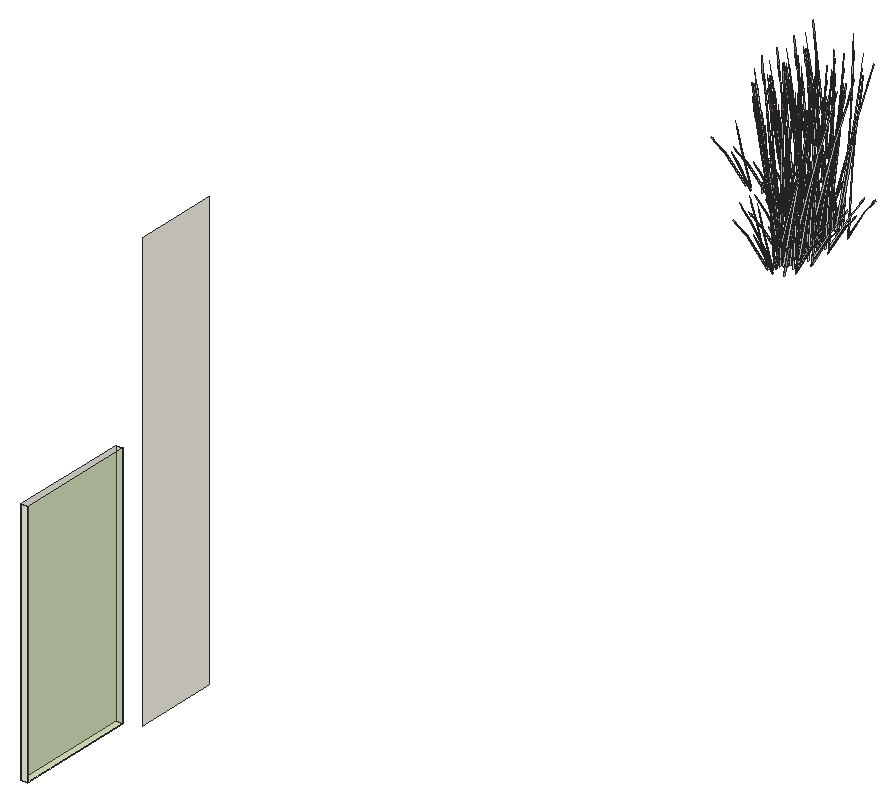
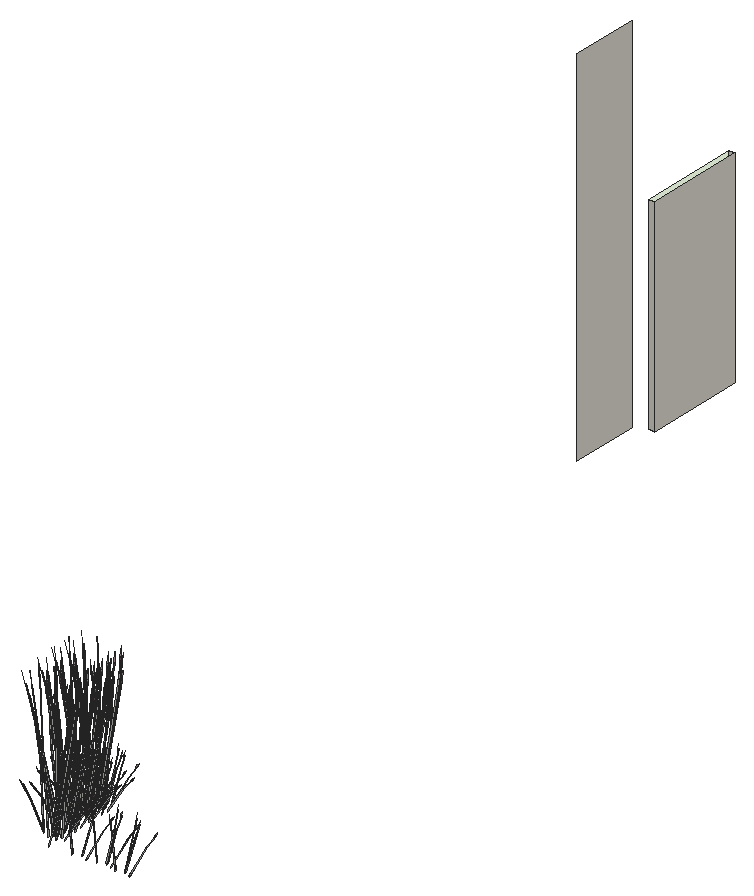
# SketchUp Ruby script. Lengths in inches.
U = 1.inch
M = Sketchup.active_model
def pt(a) = Geom::Point3d.new(a.map { |v| v * U })
def face(e, loops, mat)
  f = e.add_face(loops[0].map { |a| pt(a) })
  loops[1..].each { |l| e.add_face(l.map { |a| pt(a) }).erase! }
  f.material = f.back_material = mat if mat
  f
end
# faces: each face lists its corners as indices into pts; further lists are holes
def faces(e, pts, list, mat = nil) = list.each { |f| face(e, (f[0].is_a?(Array) ? f : [f]).map { |l| l.map { |i| pts[i] } }, mat) }
# xy, xz, yz: faces in a plane at the given z, y or x. An outline is a flat list of corners, or four numbers for a rectangle; further outlines are holes
def ring(l) = l.size == 4 ? [[l[0], l[1]], [l[2], l[1]], [l[2], l[3]], [l[0], l[3]]] : l.each_slice(2).to_a
def flat(e, list, mat, &to3) = list.each { |f| face(e, (f[0].is_a?(Array) ? f : [f]).map { |l| ring(l).map { |u, v| to3.(u, v) } }, mat) }
def xy(e, z, list, mat = nil) = flat(e, list, mat) { |x, y| [x, y, z] }
def xz(e, y, list, mat = nil) = flat(e, list, mat) { |x, z| [x, y, z] }
def yz(e, x, list, mat = nil) = flat(e, list, mat) { |y, z| [x, y, z] }
def lines(e, pts, list) = list.each { |a, b| e.add_line(pt(pts[a]), pt(pts[b])) }
# prism: a flat outline (further loops are holes) pulled along v
def prism(e, loops, v, mat = nil)
  f = face(e, loops, mat); d = Geom::Vector3d.new(v.map { |x| x * U })
  f.pushpull(f.normal.samedirection?(d) ? d.length : -d.length)
end
def box(e, o, s, mat = nil) = prism(e, [[o, [o[0] + s[0], o[1], o[2]], [o[0] + s[0], o[1] + s[1], o[2]], [o[0], o[1] + s[1], o[2]]]], [0, 0, s[2]], mat)
def at(x, y, z, deg = 0) = Geom::Transformation.translation(pt([x, y, z])) * Geom::Transformation.rotation(ORIGIN, Z_AXIS, deg.degrees)
def axes(o, x, y, z) = Geom::Transformation.new([*x, 0, *y, 0, *z, 0, *pt(o).to_a, 1])
def part(name) = M.definitions.add(name)
# library, detail: a bought-in or finely detailed component or shape, given as its bounding box
def library(name, o, s) = part(name).tap { |d| box(d.entities, o, s) }
def detail(e, o, s) = box(e.add_group.entities, o, s)
def put(e, d, t, mat = nil) = e.add_instance(d, t).tap { |i| i.material = mat if mat }
def group(e, t, mat = nil) = e.add_group.tap { |g| g.transformation = t; g.material = mat if mat }.entities
root = M.entities
M.materials.add("C01_Vanilla_Cream").color = [255, 251, 241]
M.materials.add("Glass_Basic_01").color = [119, 186, 61]
M.materials["Glass_Basic_01"].alpha = 0.25
M.materials.add("LightPink_Translucent").color = [144, 107, 117]
M.materials["LightPink_Translucent"].alpha = 0.75
c1 = part("blade")
p = [[2.15,0.21,22],[0,0.17,0],[0.09,0.45,0],[2.18,0.31,22],[2.29,0.31,22],[0.38,0.45,0],
  [2.48,0.24,33],[2.49,0.24,33],[2.48,0.22,33]]
faces(c1.entities,p,[[0,1,2,3],[4,5,2,3],[6,3,4,7],[8,0,3,6]])
c2 = part("seeds")
p = [[0.3,-0.1,1.38],[-0.01,-0.03,1.59],[-0.01,-0.03,0.03],[0.14,-0.07,-0.07],[0.29,-0.03,3],[0.15,0.01,3.11]]
faces(c2.entities,p,[[0,1,2,3],[1,0,4,5]],"LightPink_Translucent")
c3 = part("blade with seeds")
put(c3.entities,c1,at(0,0,0))
put(c3.entities,c2,axes([2.4,0.25,30.99],[1.5799,-0.05474,1.17369],[-0.12525,1.92788,0.29478],[-0.07173,-0.02425,1.56792]))
xy(root,265,[[700,25,702,59]],"C01_Vanilla_Cream")
xz(root,25,[[700,265,702,335]],"C01_Vanilla_Cream")
xz(root,59,[[700,265,702,335]],"C01_Vanilla_Cream")
yz(root,700,[[25,265,59,335]],"C01_Vanilla_Cream")
yz(root,702,[[25,265,59,335]],"Glass_Basic_01")
yz(root,706,[[61,265,84.38,389]],"C01_Vanilla_Cream")
put(root,c3,axes([687.53,307.45,265.24],[-0.10912,0.02057,1.46364],[-0.60346,-0.23156,-0.2236],[0.01013,-0.19315,0.24931]))
put(root,c3,axes([685.57,308.15,265.24],[-0.06302,0.07522,1.46364],[-0.63686,0.16217,-0.2236],[-0.15385,-0.14752,0.24931]))
put(root,c3,axes([690.2,308.43,265.24],[-0.09738,-0.04498,1.46364],[-0.25012,-0.50252,-0.2236],[0.16873,-0.13637,0.24931]))
put(root,c3,axes([687.41,307.85,265.77],[-0.44958,0.32756,-0.03231],[-0.41194,-0.35875,-0.14649],[-0.029,-0.10165,0.48318]))
put(root,c3,axes([687.03,310.37,265.83],[0.31565,-0.51449,-0.37133],[0.65588,0.24761,0.17871],[0,-0.1186,1.19224]))
put(root,c3,axes([687.32,310.12,266.21],[-0.07581,-0.65151,-0.24149],[0.7896,-0.03939,-0.41502],[0.13904,-0.08678,1.32557]))
put(root,c3,axes([685.36,310.15,265.68],[0.45414,-0.35624,-0.25712],[0.45414,0.35624,0.25712],[0,-0.11474,1.15348]))
put(root,c3,axes([685.18,308.44,265.77],[-0.18768,0.46622,-0.03231],[-0.57763,-0.14342,-0.14649],[-0.0877,-0.07626,0.48318]))
put(root,c3,axes([686.95,310.8,266.21],[-0.73268,-0.27244,-0.24149],[0.35279,-0.57501,-0.41502],[-0.02303,-0.14118,1.32557]))
put(root,c3,axes([687.22,308.67,265.68],[0.60696,0.14127,-0.25712],[-0.15283,0.49751,0.25712],[0.12236,-0.05737,1.15348]))
put(root,c3,axes([687.14,311.4,266.02],[0.17244,-0.67657,-0.19446],[0.81759,0.11793,0.42555],[-0.14286,-0.09343,1.29846]))
put(root,c3,axes([687.95,312.39,265.24],[-0.10912,0.02057,1.46364],[-0.60346,-0.23156,-0.2236],[0.01013,-0.19315,0.24931]))
put(root,c3,axes([687.08,311.13,265.83],[-0.39083,-0.47924,-0.37133],[0.59199,-0.33747,0.17871],[-0.12647,-0.0593,1.19224]))
put(root,c3,axes([691.88,310.46,265.875],[-0.40335,-0.3651,-0.05385],[0.44175,-0.33453,-0.24415],[0.12517,-0.02355,0.8053]))
put(root,c3,axes([686.57,309.7,265.32],[-0.64037,0.22859,1.07011],[-0.20382,-0.65589,0.4158],[0.39323,0.01091,1.21713]))
put(root,c3,axes([691.57,310.59,265.24],[-0.034,-0.08668,1.46364],[0.23582,-0.50706,-0.2236],[0.23788,-0.00729,0.24931]))
put(root,c3,axes([684.55,310.5,265.24],[0.0165,0.08998,1.46364],[-0.33262,0.46992,-0.2236],[-0.23626,-0.02369,0.24931]))
put(root,c3,axes([686.01,312.19,265.68],[-0.15283,-0.49751,-0.25712],[0.60696,-0.14127,0.25712],[-0.12236,-0.05737,1.15348]))
put(root,c3,axes([686,313.1,265.24],[-0.06302,0.07522,1.46364],[-0.63686,0.16217,-0.2236],[-0.15385,-0.14752,0.24931]))
put(root,c3,axes([688.23,310.03,266.21],[0.65687,-0.37907,-0.24149],[0.43681,0.53562,-0.41502],[0.16207,0.0544,1.32557]))
put(root,c3,axes([690.62,313.375,265.24],[-0.09738,-0.04498,1.46364],[-0.25012,-0.50252,-0.2236],[0.16873,-0.13637,0.24931]))
put(root,c3,axes([687.5,311.4,266.21],[-0.65687,0.37907,-0.24149],[-0.43681,-0.53562,-0.41502],[-0.16207,-0.0544,1.32557]))
put(root,c3,axes([689.72,309.24,265.68],[0.15283,0.49751,-0.25712],[-0.60696,0.14127,0.25712],[0.12236,0.05737,1.15348]))
put(root,c3,axes([687.84,312.79,265.77],[-0.44958,0.32756,-0.03231],[-0.41194,-0.35875,-0.14649],[-0.029,-0.10165,0.48318]))
put(root,c3,axes([688.63,311.96,265.8125],[0.68303,-0.19373,-0.15934],[0.24001,0.55805,0.00007],[0.07539,-0.02141,1.44335]))
put(root,c3,axes([688.24,311.57,266.05],[-0.63528,-0.45956,-0.20909],[0.53456,-0.51604,0.45758],[-0.17107,0.05376,1.39619]))
put(root,c3,axes([688.65,310.3,265.83],[0.39083,0.47924,-0.37133],[-0.59199,0.33747,0.17871],[0.12647,0.0593,1.19224]))
put(root,c3,axes([687.45,315.31,265.83],[0.31565,-0.51449,-0.37133],[0.65588,0.24761,0.17871],[0,-0.1186,1.19224]))
put(root,c3,axes([687.91,311.47,265.83],[-0.70648,0.03525,-0.37133],[-0.06389,-0.58508,0.17871],[-0.12647,0.0593,1.19224]))
put(root,c3,axes([687.74,315.06,266.21],[-0.07581,-0.65151,-0.24149],[0.7896,-0.03939,-0.41502],[0.13904,-0.08678,1.32557]))
put(root,c3,axes([685.79,315.09,265.68],[0.45414,-0.35624,-0.25712],[0.45414,0.35624,0.25712],[0,-0.11474,1.15348]))
put(root,c3,axes([685.6,313.39,265.77],[-0.18768,0.46622,-0.03231],[-0.57763,-0.14342,-0.14649],[-0.0877,-0.07626,0.48318]))
put(root,c3,axes([687.375,315.74,266.21],[-0.73268,-0.27244,-0.24149],[0.35279,-0.57501,-0.41502],[-0.02303,-0.14118,1.32557]))
put(root,c3,axes([687.64,313.62,265.68],[0.60696,0.14127,-0.25712],[-0.15283,0.49751,0.25712],[0.12236,-0.05737,1.15348]))
put(root,c3,axes([688.51,312.76,265.68],[-0.60696,-0.14127,-0.25712],[0.15283,-0.49751,0.25712],[-0.12236,0.05737,1.15348]))
put(root,c3,axes([688.78,310.63,266.21],[0.73268,0.27244,-0.24149],[-0.35279,0.57501,-0.41502],[0.02303,0.14118,1.32557]))
put(root,c3,axes([687.5625,316.35,266.02],[0.17244,-0.67657,-0.19446],[0.81759,0.11793,0.42555],[-0.14286,-0.09343,1.29846]))
put(root,c3,axes([690.37,311.28,265.68],[-0.45414,0.35624,-0.25712],[-0.45414,-0.35624,0.25712],[0,0.11474,1.15348]))
put(root,c3,axes([688.41,311.32,266.21],[0.07581,0.65151,-0.24149],[-0.7896,0.03939,-0.41502],[-0.13904,0.08678,1.32557]))
put(root,c3,axes([688.7,311.0625,265.83],[-0.31565,0.51449,-0.37133],[-0.65588,-0.24761,0.17871],[0,0.1186,1.19224]))
put(root,c3,axes([687.5,316.07,265.83],[-0.39083,-0.47924,-0.37133],[0.59199,-0.33747,0.17871],[-0.12647,-0.0593,1.19224]))
put(root,c3,axes([692.3,315.4,265.875],[-0.40335,-0.3651,-0.05385],[0.44175,-0.33453,-0.24415],[0.12517,-0.02355,0.8053]))
put(root,c3,axes([687,314.64,265.32],[-0.64037,0.22859,1.07011],[-0.20382,-0.65589,0.4158],[0.39323,0.01091,1.21713]))
put(root,c3,axes([692,315.53,265.24],[-0.034,-0.08668,1.46364],[0.23582,-0.50706,-0.2236],[0.23788,-0.00729,0.24931]))
put(root,c3,axes([689.86,313.09,265.24],[0.0474,-0.08243,1.46364],[0.59674,-0.24277,-0.2236],[0.18092,0.12565,0.24931]))
put(root,c3,axes([684.98,315.44,265.24],[0.0165,0.08998,1.46364],[-0.33262,0.46992,-0.2236],[-0.23626,-0.02369,0.24931]))
put(root,c3,axes([684.375,313.02,265.24],[0.08727,0.05704,1.46364],[0.14797,0.52853,-0.2236],[-0.19341,0.11271,0.24931]))
put(root,c3,axes([686.43,317.14,265.68],[-0.15283,-0.49751,-0.25712],[0.60696,-0.14127,0.25712],[-0.12236,-0.05737,1.15348]))
put(root,c3,axes([687.49,318.93,265.24],[-0.10912,0.02057,1.46364],[-0.60346,-0.23156,-0.2236],[0.01013,-0.19315,0.24931]))
put(root,c3,axes([688.65,314.98,266.21],[0.65687,-0.37907,-0.24149],[0.43681,0.53562,-0.41502],[0.16207,0.0544,1.32557]))
put(root,c3,axes([687.92,316.34,266.21],[-0.65687,0.37907,-0.24149],[-0.43681,-0.53562,-0.41502],[-0.16207,-0.0544,1.32557]))
put(root,c3,axes([690.14,314.18,265.68],[0.15283,0.49751,-0.25712],[-0.60696,0.14127,0.25712],[0.12236,0.05737,1.15348]))
put(root,c3,axes([689.06,316.9,265.8125],[0.68303,-0.19373,-0.15934],[0.24001,0.55805,0.00007],[0.07539,-0.02141,1.44335]))
put(root,c3,axes([687.07,313.07,265.24],[0.10529,-0.03107,1.46364],[0.63335,0.17101,-0.2236],[0.01852,0.19274,0.24931]))
put(root,c3,axes([688.66,316.51,266.05],[-0.63528,-0.45956,-0.20909],[0.53456,-0.51604,0.45758],[-0.17107,0.05376,1.39619]))
put(root,c3,axes([689.07,315.25,265.83],[0.39083,0.47924,-0.37133],[-0.59199,0.33747,0.17871],[0.12647,0.0593,1.19224]))
put(root,c3,axes([685.54,319.64,265.24],[-0.06302,0.07522,1.46364],[-0.63686,0.16217,-0.2236],[-0.15385,-0.14752,0.24931]))
put(root,c3,axes([690.16,319.92,265.24],[-0.09738,-0.04498,1.46364],[-0.25012,-0.50252,-0.2236],[0.16873,-0.13637,0.24931]))
put(root,c3,axes([688.34,316.42,265.83],[-0.70648,0.03525,-0.37133],[-0.06389,-0.58508,0.17871],[-0.12647,0.0593,1.19224]))
put(root,c3,axes([687.38,319.33,265.77],[-0.44958,0.32756,-0.03231],[-0.41194,-0.35875,-0.14649],[-0.029,-0.10165,0.48318]))
put(root,c3,axes([688.9375,317.7,265.68],[-0.60696,-0.14127,-0.25712],[0.15283,-0.49751,0.25712],[-0.12236,0.05737,1.15348]))
put(root,c3,axes([689.2,315.58,266.21],[0.73268,0.27244,-0.24149],[-0.35279,0.57501,-0.41502],[0.02303,0.14118,1.32557]))
put(root,c3,axes([690.79,316.22,265.68],[-0.45414,0.35624,-0.25712],[-0.45414,-0.35624,0.25712],[0,0.11474,1.15348]))
put(root,c3,axes([688.83,316.26,266.21],[0.07581,0.65151,-0.24149],[-0.7896,0.03939,-0.41502],[-0.13904,0.08678,1.32557]))
put(root,c3,axes([689.12,316,265.83],[-0.31565,0.51449,-0.37133],[-0.65588,-0.24761,0.17871],[0,0.1186,1.19224]))
put(root,c3,axes([687.29,321.6,266.21],[-0.07581,-0.65151,-0.24149],[0.7896,-0.03939,-0.41502],[0.13904,-0.08678,1.32557]))
put(root,c3,axes([685.33,321.64,265.68],[0.45414,-0.35624,-0.25712],[0.45414,0.35624,0.25712],[0,-0.11474,1.15348]))
put(root,c3,axes([685.15,319.93,265.77],[-0.18768,0.46622,-0.03231],[-0.57763,-0.14342,-0.14649],[-0.0877,-0.07626,0.48318]))
put(root,c3,axes([686.92,322.28,266.21],[-0.73268,-0.27244,-0.24149],[0.35279,-0.57501,-0.41502],[-0.02303,-0.14118,1.32557]))
put(root,c3,axes([687.18,320.16,265.68],[0.60696,0.14127,-0.25712],[-0.15283,0.49751,0.25712],[0.12236,-0.05737,1.15348]))
put(root,c3,axes([690.28,318.03,265.24],[0.0474,-0.08243,1.46364],[0.59674,-0.24277,-0.2236],[0.18092,0.12565,0.24931]))
put(root,c3,axes([684.8,317.96,265.24],[0.08727,0.05704,1.46364],[0.14797,0.52853,-0.2236],[-0.19341,0.11271,0.24931]))
put(root,c3,axes([687.1,322.89,266.02],[0.17244,-0.67657,-0.19446],[0.81759,0.11793,0.42555],[-0.14286,-0.09343,1.29846]))
put(root,c3,axes([687.05,322.61,265.83],[-0.39083,-0.47924,-0.37133],[0.59199,-0.33747,0.17871],[-0.12647,-0.0593,1.19224]))
put(root,c3,axes([691.85,321.94,265.875],[-0.40335,-0.3651,-0.05385],[0.44175,-0.33453,-0.24415],[0.12517,-0.02355,0.8053]))
put(root,c3,axes([687.49,318.01,265.24],[0.10529,-0.03107,1.46364],[0.63335,0.17101,-0.2236],[0.01852,0.19274,0.24931]))
put(root,c3,axes([686.54,321.18,265.32],[-0.64037,0.22859,1.07011],[-0.20382,-0.65589,0.4158],[0.39323,0.01091,1.21713]))
put(root,c3,axes([691.54,322.07,265.24],[-0.034,-0.08668,1.46364],[0.23582,-0.50706,-0.2236],[0.23788,-0.00729,0.24931]))
put(root,c3,axes([684.52,321.98,265.24],[0.0165,0.08998,1.46364],[-0.33262,0.46992,-0.2236],[-0.23626,-0.02369,0.24931]))
put(root,c3,axes([685.98,323.68,265.68],[-0.15283,-0.49751,-0.25712],[0.60696,-0.14127,0.25712],[-0.12236,-0.05737,1.15348]))
put(root,c3,axes([688.2,321.52,266.21],[0.65687,-0.37907,-0.24149],[0.43681,0.53562,-0.41502],[0.16207,0.0544,1.32557]))
put(root,c3,axes([687.46,322.88,266.21],[-0.65687,0.37907,-0.24149],[-0.43681,-0.53562,-0.41502],[-0.16207,-0.0544,1.32557]))
put(root,c3,axes([689.68,320.72,265.68],[0.15283,0.49751,-0.25712],[-0.60696,0.14127,0.25712],[0.12236,0.05737,1.15348]))
put(root,c3,axes([688.6,323.45,265.8125],[0.68303,-0.19373,-0.15934],[0.24001,0.55805,0.00007],[0.07539,-0.02141,1.44335]))
put(root,c3,axes([688.2,323.06,266.05],[-0.63528,-0.45956,-0.20909],[0.53456,-0.51604,0.45758],[-0.17107,0.05376,1.39619]))
put(root,c3,axes([686.4375,327.13,265.24],[-0.10912,0.02057,1.46364],[-0.60346,-0.23156,-0.2236],[0.01013,-0.19315,0.24931]))
put(root,c3,axes([688.61,321.79,265.83],[0.39083,0.47924,-0.37133],[-0.59199,0.33747,0.17871],[0.12647,0.0593,1.19224]))
put(root,c3,axes([687.88,322.96,265.83],[-0.70648,0.03525,-0.37133],[-0.06389,-0.58508,0.17871],[-0.12647,0.0593,1.19224]))
put(root,c3,axes([688.48,324.24,265.68],[-0.60696,-0.14127,-0.25712],[0.15283,-0.49751,0.25712],[-0.12236,0.05737,1.15348]))
put(root,c3,axes([688.74,322.12,266.21],[0.73268,0.27244,-0.24149],[-0.35279,0.57501,-0.41502],[0.02303,0.14118,1.32557]))
put(root,c3,axes([690.33,322.76,265.68],[-0.45414,0.35624,-0.25712],[-0.45414,-0.35624,0.25712],[0,0.11474,1.15348]))
put(root,c3,axes([684.49,327.84,265.24],[-0.06302,0.07522,1.46364],[-0.63686,0.16217,-0.2236],[-0.15385,-0.14752,0.24931]))
put(root,c3,axes([688.375,322.8,266.21],[0.07581,0.65151,-0.24149],[-0.7896,0.03939,-0.41502],[-0.13904,0.08678,1.32557]))
put(root,c3,axes([688.66,322.54,265.83],[-0.31565,0.51449,-0.37133],[-0.65588,-0.24761,0.17871],[0,0.1186,1.19224]))
put(root,c3,axes([689.11,328.12,265.24],[-0.09738,-0.04498,1.46364],[-0.25012,-0.50252,-0.2236],[0.16873,-0.13637,0.24931]))
put(root,c3,axes([686.33,327.53,265.77],[-0.44958,0.32756,-0.03231],[-0.41194,-0.35875,-0.14649],[-0.029,-0.10165,0.48318]))
put(root,c3,axes([689.82,324.57,265.24],[0.0474,-0.08243,1.46364],[0.59674,-0.24277,-0.2236],[0.18092,0.12565,0.24931]))
put(root,c3,axes([684.34,324.5,265.24],[0.08727,0.05704,1.46364],[0.14797,0.52853,-0.2236],[-0.19341,0.11271,0.24931]))
put(root,c3,axes([686.23,329.8,266.21],[-0.07581,-0.65151,-0.24149],[0.7896,-0.03939,-0.41502],[0.13904,-0.08678,1.32557]))
put(root,c3,axes([684.27,329.84,265.68],[0.45414,-0.35624,-0.25712],[0.45414,0.35624,0.25712],[0,-0.11474,1.15348]))
put(root,c3,axes([684.09,328.13,265.77],[-0.18768,0.46622,-0.03231],[-0.57763,-0.14342,-0.14649],[-0.0877,-0.07626,0.48318]))
put(root,c3,axes([685.86,330.48,266.21],[-0.73268,-0.27244,-0.24149],[0.35279,-0.57501,-0.41502],[-0.02303,-0.14118,1.32557]))
put(root,c3,axes([686.13,328.36,265.68],[0.60696,0.14127,-0.25712],[-0.15283,0.49751,0.25712],[0.12236,-0.05737,1.15348]))
put(root,c3,axes([687.04,324.55,265.24],[0.10529,-0.03107,1.46364],[0.63335,0.17101,-0.2236],[0.01852,0.19274,0.24931]))
put(root,c3,axes([686.05,331.09,266.02],[0.17244,-0.67657,-0.19446],[0.81759,0.11793,0.42555],[-0.14286,-0.09343,1.29846]))
put(root,c3,axes([690.79,330.14,265.875],[-0.40335,-0.3651,-0.05385],[0.44175,-0.33453,-0.24415],[0.12517,-0.02355,0.8053]))
put(root,c3,axes([666.97,333.2,265.24],[-0.10912,0.02057,1.46364],[-0.60346,-0.23156,-0.2236],[0.01013,-0.19315,0.24931]))
put(root,c3,axes([685.48,329.38,265.32],[-0.64037,0.22859,1.07011],[-0.20382,-0.65589,0.4158],[0.39323,0.01091,1.21713]))
put(root,c3,axes([690.49,330.27,265.24],[-0.034,-0.08668,1.46364],[0.23582,-0.50706,-0.2236],[0.23788,-0.00729,0.24931]))
put(root,c3,axes([683.47,330.18,265.24],[0.0165,0.08998,1.46364],[-0.33262,0.46992,-0.2236],[-0.23626,-0.02369,0.24931]))
put(root,c3,axes([684.92,331.88,265.68],[-0.15283,-0.49751,-0.25712],[0.60696,-0.14127,0.25712],[-0.12236,-0.05737,1.15348]))
put(root,c3,axes([660.27,333.73,265.24],[-0.10912,0.02057,1.46364],[-0.60346,-0.23156,-0.2236],[0.01013,-0.19315,0.24931]))
put(root,c3,axes([687.14,329.72,266.21],[0.65687,-0.37907,-0.24149],[0.43681,0.53562,-0.41502],[0.16207,0.0544,1.32557]))
put(root,c3,axes([674.87,333.79,265.24],[-0.10912,0.02057,1.46364],[-0.60346,-0.23156,-0.2236],[0.01013,-0.19315,0.24931]))
put(root,c3,axes([686.41,331.08,266.21],[-0.65687,0.37907,-0.24149],[-0.43681,-0.53562,-0.41502],[-0.16207,-0.0544,1.32557]))
put(root,c3,axes([688.63,328.92,265.68],[0.15283,0.49751,-0.25712],[-0.60696,0.14127,0.25712],[0.12236,0.05737,1.15348]))
put(root,c3,axes([687.55,331.65,265.8125],[0.68303,-0.19373,-0.15934],[0.24001,0.55805,0.00007],[0.07539,-0.02141,1.44335]))
put(root,c3,axes([665.02,333.9,265.24],[-0.06302,0.07522,1.46364],[-0.63686,0.16217,-0.2236],[-0.15385,-0.14752,0.24931]))
put(root,c3,axes([687.15,331.26,266.05],[-0.63528,-0.45956,-0.20909],[0.53456,-0.51604,0.45758],[-0.17107,0.05376,1.39619]))
put(root,c3,axes([669.64,334.18,265.24],[-0.09738,-0.04498,1.46364],[-0.25012,-0.50252,-0.2236],[0.16873,-0.13637,0.24931]))
put(root,c3,axes([685.1,335.32,265.24],[-0.10912,0.02057,1.46364],[-0.60346,-0.23156,-0.2236],[0.01013,-0.19315,0.24931]))
put(root,c3,axes([658.32,334.4375,265.24],[-0.06302,0.07522,1.46364],[-0.63686,0.16217,-0.2236],[-0.15385,-0.14752,0.24931]))
put(root,c3,axes([672.92,334.5,265.24],[-0.06302,0.07522,1.46364],[-0.63686,0.16217,-0.2236],[-0.15385,-0.14752,0.24931]))
put(root,c3,axes([662.9375,334.72,265.24],[-0.09738,-0.04498,1.46364],[-0.25012,-0.50252,-0.2236],[0.16873,-0.13637,0.24931]))
put(root,c3,axes([677.54,334.78,265.24],[-0.09738,-0.04498,1.46364],[-0.25012,-0.50252,-0.2236],[0.16873,-0.13637,0.24931]))
put(root,c3,axes([666.86,333.6,265.77],[-0.44958,0.32756,-0.03231],[-0.41194,-0.35875,-0.14649],[-0.029,-0.10165,0.48318]))
put(root,c3,axes([660.15,334.13,265.77],[-0.44958,0.32756,-0.03231],[-0.41194,-0.35875,-0.14649],[-0.029,-0.10165,0.48318]))
